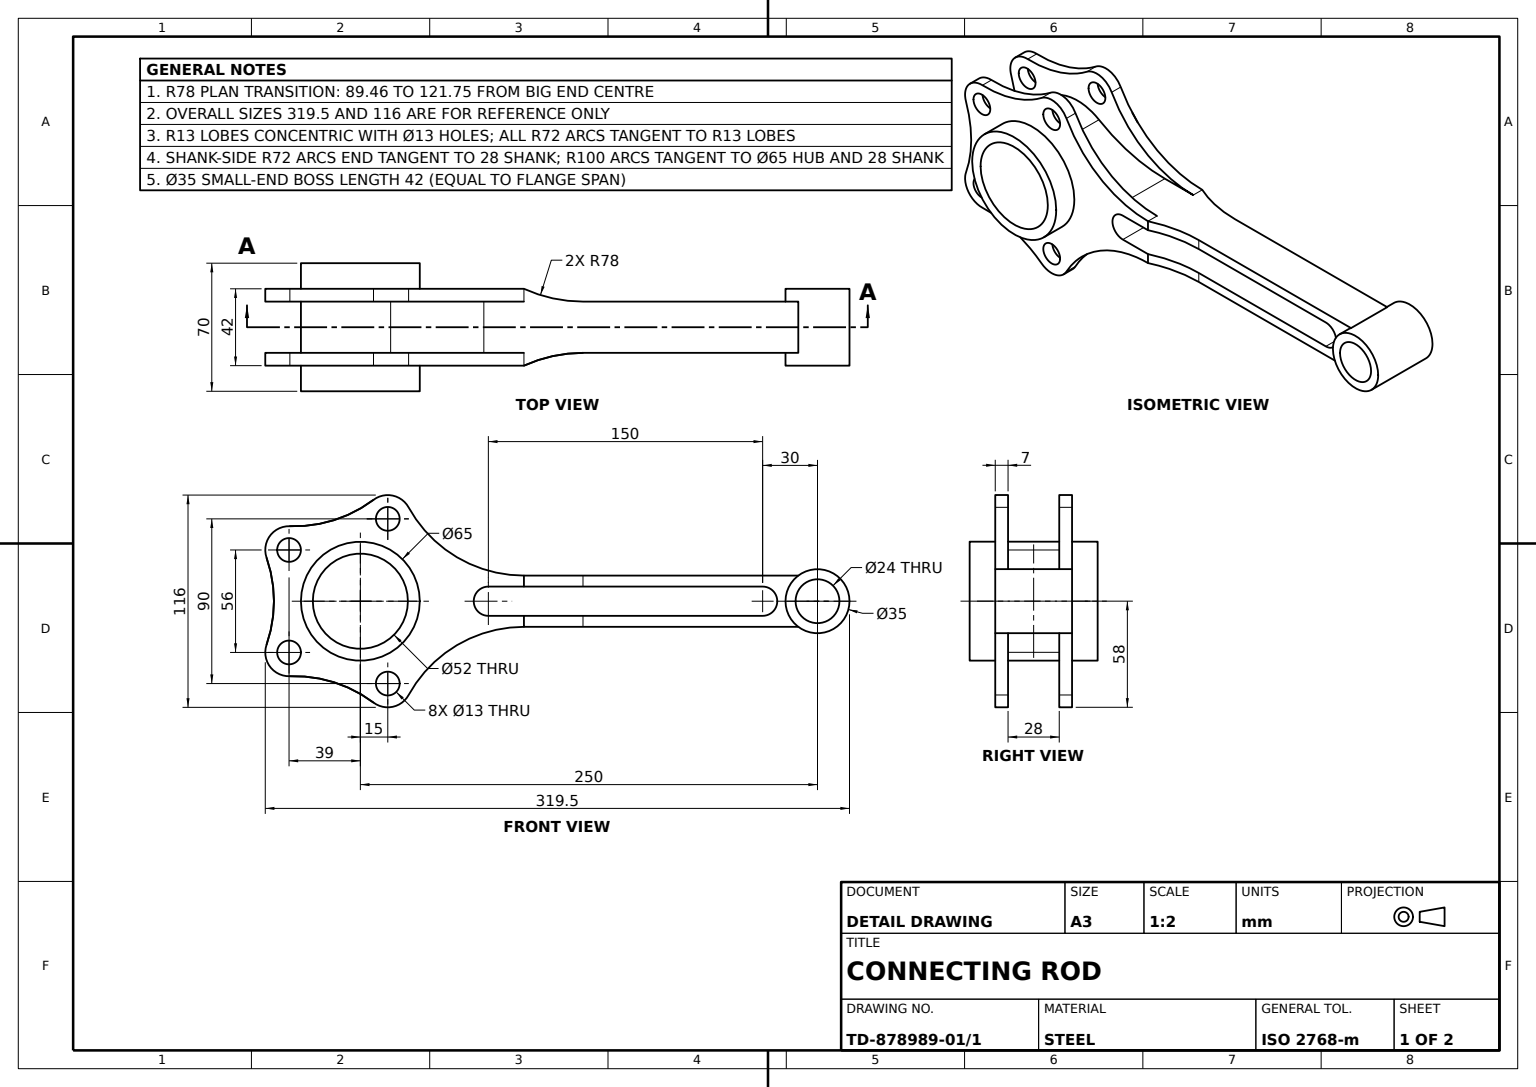
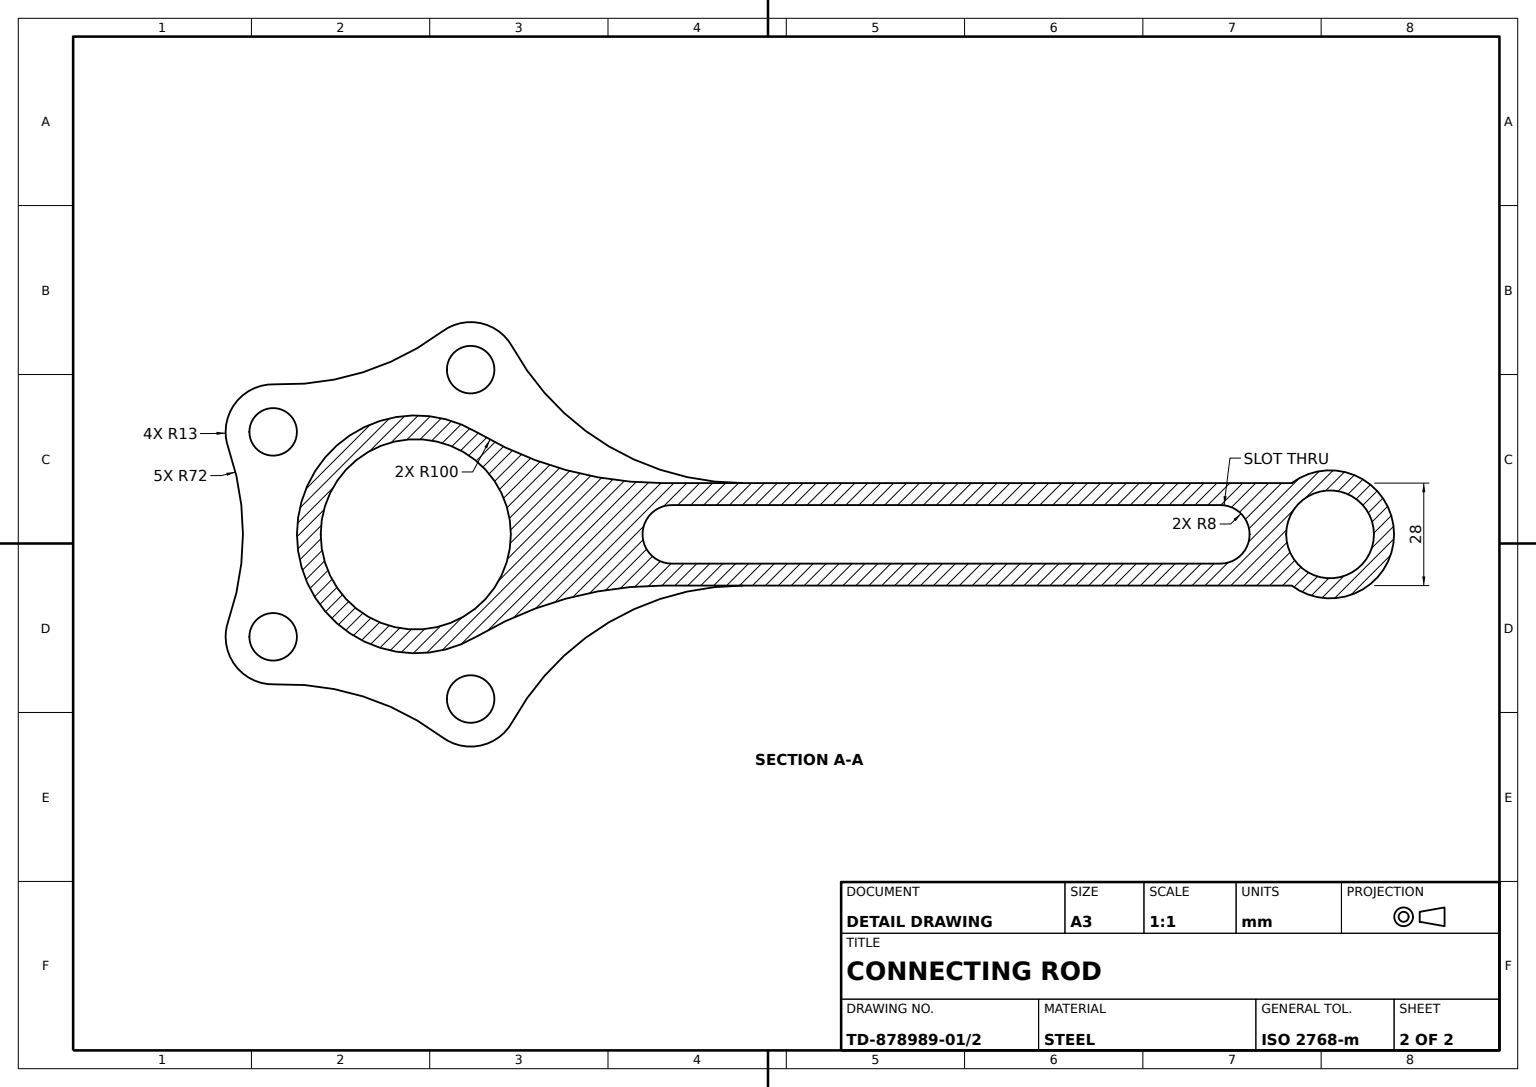
solid
v1 (8.5,-45,14)
v2 (8.5,-45,21)
e1 v1 v2 LINE
v3 (21.5,-45,14)
e2 v1 v3 CIRCLE(AX(P(15,-45,14),D(0,0,-1),D(1,0,0)),6.5)
v4 (21.5,-45,21)
e3 v3 v4 LINE
e4 v2 v4 CIRCLE(AX(P(15,-45,21),D(0,0,-1),D(1,0,0)),6.5)
face CYL(AX(P(15,-45,14),D(0,0,1),D(1,0,0)),6.5) rev [-e1 e2 e3 -e4]
v5 (67.529623,14,14)
v6 (89.458042,14,14)
e5 v5 v6 LINE
v7 (89.458042,14,21)
e6 v6 v7 LINE
v8 (121.753552,14,14)
e7 v7 v8 CIRCLE(AX(P(121.753552,14,92),D(0,-1,0),D(-1,0,0)),78)
v9 (239.5,14,14)
e8 v8 v9 LINE
v10 (239.5,14,-14)
e9 v9 v10 LINE
v11 (121.753552,14,-14)
e10 v11 v10 LINE
v12 (89.458042,14,-21)
e11 v11 v12 CIRCLE(AX(P(121.753552,14,-92),D(0,-1,0),D(-1,0,0)),78)
v13 (89.458042,14,-14)
e12 v13 v12 LINE
v14 (67.529623,14,-14)
e13 v14 v13 LINE
e14 v5 v14 LINE
face PLANE(AX(P(67.529623,14,14),D(0,1,0),D(-1,0,0))) [e5 e6 e7 e8 e9 -e10 e11 -e12 -e13 -e14]
v15 (89.458042,8,-21)
e15 v12 v15 LINE
v16 (121.753552,8,-14)
e16 v16 v11 LINE
e17 v15 v16 CIRCLE(AX(P(121.753552,8,-92),D(0,1,0),D(0,0,1)),78)
face CYL(AX(P(121.753552,14,-92),D(0,1,0),D(0,0,1)),78) rev [-e15 -e11 -e16 -e17]
v17 (8.5,45,14)
v18 (8.5,45,21)
e18 v17 v18 LINE
v19 (21.5,45,21)
e19 v18 v19 CIRCLE(AX(P(15,45,21),D(0,0,1),D(1,0,0)),6.5)
v20 (21.5,45,14)
e20 v20 v19 LINE
e21 v17 v20 CIRCLE(AX(P(15,45,14),D(0,0,1),D(1,0,0)),6.5)
face CYL(AX(P(15,45,14),D(0,0,1),D(1,0,0)),6.5) rev [e18 e19 -e20 -e21]
v21 (-38.551485,40.992261,-21)
v22 (7.189691,55.392261,-21)
e22 v21 v22 CIRCLE(AX(P(-36.067402,112.949396,-21),D(0,0,1),D(1,0,0)),72)
v23 (-38.551485,40.992261,-14)
e23 v23 v21 LINE
v24 (7.189691,55.392261,-14)
e24 v23 v24 CIRCLE(AX(P(-36.067402,112.949396,-14),D(0,0,1),D(1,0,0)),72)
e25 v24 v22 LINE
face CYL(AX(P(-36.067402,112.949396,-14),D(0,0,-1),D(-1,0,0)),72) rev [-e22 -e23 e24 e25]
v25 (-38.551485,-40.992261,14)
v26 (-51.274423,-23.717647,14)
e26 v25 v26 CIRCLE(AX(P(-39,-28,14),D(0,0,-1),D(-1,0,0)),13)
v27 (-38.551485,-40.992261,21)
e27 v25 v27 LINE
v28 (-51.274423,-23.717647,21)
e28 v27 v28 CIRCLE(AX(P(-39,-28,21),D(0,0,-1),D(-1,0,0)),13)
e29 v26 v28 LINE
face CYL(AX(P(-39,-28,14),D(0,0,1),D(1,0,0)),13) [-e26 e27 e28 -e29]
v29 (121.753552,8,14)
v30 (89.458042,8,21)
e30 v29 v30 CIRCLE(AX(P(121.753552,8,92),D(0,1,0),D(0,0,1)),78)
e31 v8 v29 LINE
e32 v7 v30 LINE
face CYL(AX(P(121.753552,14,92),D(0,1,0),D(0,0,1)),78) rev [-e30 -e31 -e7 e32]
v31 (26.387701,-51.270588,14)
v32 (89.458042,-14,14)
e33 v31 v32 CIRCLE(AX(P(89.458042,-86,14),D(0,0,-1),D(-1,0,0)),72)
v33 (7.189691,-55.392261,14)
e34 v31 v33 CIRCLE(AX(P(15,-45,14),D(0,0,-1),D(-1,0,0)),13)
e35 v25 v33 CIRCLE(AX(P(-36.067402,-112.949396,14),D(0,0,-1),D(-1,0,0)),72)
v34 (-47.255841,0,14)
e36 v26 v34 CIRCLE(AX(P(-119.255841,0,14),D(0,0,1),D(1,0,0)),72)
v35 (-51.274423,23.717647,14)
e37 v34 v35 CIRCLE(AX(P(-119.255841,0,14),D(0,0,1),D(1,0,0)),72)
v36 (-38.551485,40.992261,14)
e38 v36 v35 CIRCLE(AX(P(-39,28,14),D(0,0,1),D(1,0,0)),13)
v37 (7.189691,55.392261,14)
e39 v36 v37 CIRCLE(AX(P(-36.067402,112.949396,14),D(0,0,1),D(1,0,0)),72)
v38 (26.387701,51.270588,14)
e40 v38 v37 CIRCLE(AX(P(15,45,14),D(0,0,1),D(1,0,0)),13)
e41 v38 v6 CIRCLE(AX(P(89.458042,86,14),D(0,0,1),D(1,0,0)),72)
v39 (16.56387,27.962264,14)
e42 v39 v5 CIRCLE(AX(P(67.529623,114,14),D(0,0,1),D(1,0,0)),100)
v40 (-32.5,0,14)
e43 v39 v40 CIRCLE(AX(P(0,0,14),D(0,0,1),D(1,0,0)),32.5)
v41 (16.56387,-27.962264,14)
e44 v40 v41 CIRCLE(AX(P(0,0,14),D(0,0,1),D(1,0,0)),32.5)
v42 (67.529623,-14,14)
e45 v41 v42 CIRCLE(AX(P(67.529623,-114,14),D(0,0,-1),D(-1,0,0)),100)
e46 v42 v32 LINE
e47 v20 v17 CIRCLE(AX(P(15,45,14),D(0,0,1),D(1,0,0)),6.5)
v43 (-32.5,28,14)
v44 (-45.5,28,14)
e48 v43 v44 CIRCLE(AX(P(-39,28,14),D(0,0,1),D(1,0,0)),6.5)
e49 v44 v43 CIRCLE(AX(P(-39,28,14),D(0,0,1),D(1,0,0)),6.5)
e50 v3 v1 CIRCLE(AX(P(15,-45,14),D(0,0,-1),D(1,0,0)),6.5)
v45 (-32.5,-28,14)
v46 (-45.5,-28,14)
e51 v45 v46 CIRCLE(AX(P(-39,-28,14),D(0,0,-1),D(1,0,0)),6.5)
e52 v46 v45 CIRCLE(AX(P(-39,-28,14),D(0,0,-1),D(1,0,0)),6.5)
face PLANE(AX(P(-39,28,14),D(0,0,1),D(1,0,0))) rev [-e33 e34 -e35 e26 e36 e37 -e38 e39 -e40 e41 -e5 -e42 e43 e44 e45 e46] [e21 e47] [e48 e49] [-e2 -e50] [-e51 -e52]
v47 (-45.5,28,-21)
v48 (-32.5,28,-21)
e53 v47 v48 CIRCLE(AX(P(-39,28,-21),D(0,0,1),D(1,0,0)),6.5)
e54 v48 v47 CIRCLE(AX(P(-39,28,-21),D(0,0,1),D(1,0,0)),6.5)
v49 (-32.5,-28,-21)
v50 (-45.5,-28,-21)
e55 v49 v50 CIRCLE(AX(P(-39,-28,-21),D(0,0,-1),D(1,0,0)),6.5)
e56 v50 v49 CIRCLE(AX(P(-39,-28,-21),D(0,0,-1),D(1,0,0)),6.5)
v51 (-32.5,0,-21)
v52 (32.5,0,-21)
e57 v51 v52 CIRCLE(AX(P(0,0,-21),D(0,0,-1),D(-1,0,0)),32.5)
e58 v52 v51 CIRCLE(AX(P(0,0,-21),D(0,0,-1),D(-1,0,0)),32.5)
v53 (-52,28,-21)
e59 v21 v53 CIRCLE(AX(P(-39,28,-21),D(0,0,1),D(1,0,0)),13)
v54 (26.387701,51.270588,-21)
e60 v54 v22 CIRCLE(AX(P(15,45,-21),D(0,0,1),D(1,0,0)),13)
e61 v54 v12 CIRCLE(AX(P(89.458042,86,-21),D(0,0,1),D(1,0,0)),72)
v55 (70,8,-21)
e62 v55 v15 LINE
v56 (70,-8,-21)
e63 v56 v55 CIRCLE(AX(P(70,0,-21),D(0,0,-1),D(-1,0,0)),8)
v57 (89.458042,-8,-21)
e64 v57 v56 LINE
v58 (89.458042,-14,-21)
e65 v57 v58 LINE
v59 (26.387701,-51.270588,-21)
e66 v59 v58 CIRCLE(AX(P(89.458042,-86,-21),D(0,0,-1),D(-1,0,0)),72)
v60 (7.189691,-55.392261,-21)
e67 v59 v60 CIRCLE(AX(P(15,-45,-21),D(0,0,-1),D(-1,0,0)),13)
v61 (-38.551485,-40.992261,-21)
e68 v61 v60 CIRCLE(AX(P(-36.067402,-112.949396,-21),D(0,0,-1),D(-1,0,0)),72)
v62 (-52,-28,-21)
e69 v61 v62 CIRCLE(AX(P(-39,-28,-21),D(0,0,-1),D(-1,0,0)),13)
v63 (-51.274423,-23.717647,-21)
e70 v62 v63 CIRCLE(AX(P(-39,-28,-21),D(0,0,-1),D(-1,0,0)),13)
v64 (-51.274423,23.717647,-21)
e71 v63 v64 CIRCLE(AX(P(-119.255841,0,-21),D(0,0,1),D(1,0,0)),72)
e72 v53 v64 CIRCLE(AX(P(-39,28,-21),D(0,0,1),D(1,0,0)),13)
v65 (8.5,-45,-21)
v66 (21.5,-45,-21)
e73 v65 v66 CIRCLE(AX(P(15,-45,-21),D(0,0,-1),D(1,0,0)),6.5)
e74 v66 v65 CIRCLE(AX(P(15,-45,-21),D(0,0,-1),D(1,0,0)),6.5)
v67 (8.5,45,-21)
v68 (21.5,45,-21)
e75 v67 v68 CIRCLE(AX(P(15,45,-21),D(0,0,1),D(1,0,0)),6.5)
e76 v68 v67 CIRCLE(AX(P(15,45,-21),D(0,0,1),D(1,0,0)),6.5)
face PLANE(AX(P(-39,28,-21),D(0,0,-1),D(1,0,0))) [e53 e54] [-e55 -e56] [-e57 -e58] [-e59 e22 -e60 e61 e15 -e62 -e63 -e64 e65 -e66 e67 -e68 e69 e70 e71 -e72] [-e73 -e74] [e75 e76]
v69 (8.5,45,-14)
e77 v69 v67 LINE
v70 (21.5,45,-14)
e78 v70 v68 LINE
e79 v70 v69 CIRCLE(AX(P(15,45,-14),D(0,0,1),D(1,0,0)),6.5)
face CYL(AX(P(15,45,-14),D(0,0,-1),D(-1,0,0)),6.5) rev [e77 -e76 -e78 e79]
v71 (-45.5,28,-14)
e80 v71 v47 LINE
v72 (-32.5,28,-14)
e81 v72 v48 LINE
e82 v72 v71 CIRCLE(AX(P(-39,28,-14),D(0,0,1),D(1,0,0)),6.5)
face CYL(AX(P(-39,28,-14),D(0,0,-1),D(-1,0,0)),6.5) rev [e80 -e54 -e81 e82]
v73 (70,8,21)
e83 v55 v73 LINE
v74 (70,-8,21)
e84 v73 v74 CIRCLE(AX(P(70,0,21),D(0,0,1),D(1,0,0)),8)
e85 v56 v74 LINE
face CYL(AX(P(70,0,-25),D(0,0,1),D(1,0,0)),8) rev [e63 e83 e84 -e85]
v75 (-38.551485,40.992261,21)
v76 (7.189691,55.392261,21)
e86 v75 v76 CIRCLE(AX(P(-36.067402,112.949396,21),D(0,0,1),D(1,0,0)),72)
e87 v37 v76 LINE
e88 v36 v75 LINE
face CYL(AX(P(-36.067402,112.949396,14),D(0,0,1),D(1,0,0)),72) rev [e86 -e87 -e39 e88]
v77 (7.189691,-55.392261,-14)
e89 v77 v60 LINE
v78 (26.387701,-51.270588,-14)
e90 v78 v59 LINE
e91 v78 v77 CIRCLE(AX(P(15,-45,-14),D(0,0,-1),D(-1,0,0)),13)
face CYL(AX(P(15,-45,-14),D(0,0,-1),D(-1,0,0)),13) [e89 -e67 -e90 e91]
v79 (-47.255841,0,21)
e92 v28 v79 CIRCLE(AX(P(-119.255841,0,21),D(0,0,1),D(1,0,0)),72)
v80 (7.189691,-55.392261,21)
e93 v27 v80 CIRCLE(AX(P(-36.067402,-112.949396,21),D(0,0,-1),D(-1,0,0)),72)
v81 (26.387701,-51.270588,21)
e94 v81 v80 CIRCLE(AX(P(15,-45,21),D(0,0,-1),D(-1,0,0)),13)
v82 (89.458042,-14,21)
e95 v81 v82 CIRCLE(AX(P(89.458042,-86,21),D(0,0,-1),D(-1,0,0)),72)
v83 (89.458042,-8,21)
e96 v83 v82 LINE
e97 v74 v83 LINE
e98 v30 v73 LINE
v84 (26.387701,51.270588,21)
e99 v84 v7 CIRCLE(AX(P(89.458042,86,21),D(0,0,1),D(1,0,0)),72)
e100 v84 v76 CIRCLE(AX(P(15,45,21),D(0,0,1),D(1,0,0)),13)
v85 (-51.274423,23.717647,21)
e101 v75 v85 CIRCLE(AX(P(-39,28,21),D(0,0,1),D(1,0,0)),13)
e102 v79 v85 CIRCLE(AX(P(-119.255841,0,21),D(0,0,1),D(1,0,0)),72)
v86 (-32.5,28,21)
v87 (-45.5,28,21)
e103 v86 v87 CIRCLE(AX(P(-39,28,21),D(0,0,1),D(1,0,0)),6.5)
e104 v87 v86 CIRCLE(AX(P(-39,28,21),D(0,0,1),D(1,0,0)),6.5)
v88 (-32.5,0,21)
v89 (32.5,0,21)
e105 v88 v89 CIRCLE(AX(P(0,0,21),D(0,0,1),D(1,0,0)),32.5)
e106 v89 v88 CIRCLE(AX(P(0,0,21),D(0,0,1),D(1,0,0)),32.5)
v90 (-45.5,-28,21)
v91 (-32.5,-28,21)
e107 v90 v91 CIRCLE(AX(P(-39,-28,21),D(0,0,-1),D(1,0,0)),6.5)
e108 v91 v90 CIRCLE(AX(P(-39,-28,21),D(0,0,-1),D(1,0,0)),6.5)
e109 v19 v18 CIRCLE(AX(P(15,45,21),D(0,0,1),D(1,0,0)),6.5)
e110 v4 v2 CIRCLE(AX(P(15,-45,21),D(0,0,-1),D(1,0,0)),6.5)
face PLANE(AX(P(-39,28,21),D(0,0,1),D(1,0,0))) [-e92 -e28 e93 -e94 e95 -e96 -e97 -e84 -e98 -e32 -e99 e100 -e86 e101 -e102] [-e103 -e104] [-e105 -e106] [e107 e108] [-e109 -e19] [e110 e4]
e111 v44 v87 LINE
e112 v43 v86 LINE
face CYL(AX(P(-39,28,14),D(0,0,1),D(1,0,0)),6.5) rev [e103 -e111 -e48 e112]
v92 (238,0,21)
v93 (262,0,21)
e113 v92 v93 CIRCLE(AX(P(250,0,21),D(0,0,1),D(1,0,0)),12)
v94 (262,0,-21)
e114 v93 v94 LINE
v95 (238,0,-21)
e115 v95 v94 CIRCLE(AX(P(250,0,-21),D(0,0,1),D(1,0,0)),12)
e116 v92 v95 LINE
face CYL(AX(P(250,0,21),D(0,0,-1),D(-1,0,0)),12) rev [e113 e114 -e115 -e116]
v96 (-52,28,-14)
v97 (-51.274423,23.717647,-14)
e117 v96 v97 CIRCLE(AX(P(-39,28,-14),D(0,0,1),D(1,0,0)),13)
e118 v96 v53 LINE
e119 v97 v64 LINE
face CYL(AX(P(-39,28,-14),D(0,0,-1),D(-1,0,0)),13) [-e117 e118 e72 -e119]
v98 (-32.5,0,35)
v99 (32.5,0,35)
e120 v98 v99 CIRCLE(AX(P(0,0,35),D(0,0,1),D(1,0,0)),32.5)
e121 v99 v98 CIRCLE(AX(P(0,0,35),D(0,0,1),D(1,0,0)),32.5)
v100 (26,0,35)
v101 (-26,0,35)
e122 v100 v101 CIRCLE(AX(P(0,0,35),D(0,0,1),D(1,0,0)),26)
e123 v101 v100 CIRCLE(AX(P(0,0,35),D(0,0,1),D(1,0,0)),26)
face PLANE(AX(P(0,0,35),D(0,0,1),D(1,0,0))) [e120 e121] [-e122 -e123]
v102 (220,8,-14)
e124 v102 v16 LINE
v103 (220,8,14)
e125 v102 v103 LINE
e126 v103 v29 LINE
face PLANE(AX(P(70,8,-25),D(0,1,0),D(0,0,1))) rev [e17 -e124 e125 e126 e30 e98 -e83 e62]
v104 (228,0,-14)
e127 v104 v102 CIRCLE(AX(P(220,0,-14),D(0,0,1),D(1,0,0)),8)
v105 (228,0,14)
e128 v104 v105 LINE
e129 v105 v103 CIRCLE(AX(P(220,0,14),D(0,0,1),D(1,0,0)),8)
face CYL(AX(P(220,0,-25),D(0,0,1),D(1,0,0)),8) rev [-e125 -e127 e128 e129]
v106 (121.753552,-8,-14)
e130 v106 v57 CIRCLE(AX(P(121.753552,-8,-92),D(0,-1,0),D(0,0,-1)),78)
v107 (121.753552,-14,-14)
e131 v107 v106 LINE
e132 v58 v107 CIRCLE(AX(P(121.753552,-14,-92),D(0,1,0),D(-1,0,0)),78)
face CYL(AX(P(121.753552,14,-92),D(0,1,0),D(0,0,1)),78) rev [-e65 -e130 -e131 -e132]
v108 (-51.274423,-23.717647,-14)
e133 v108 v97 CIRCLE(AX(P(-119.255841,0,-14),D(0,0,1),D(1,0,0)),72)
e134 v108 v63 LINE
face CYL(AX(P(-119.255841,0,-14),D(0,0,-1),D(-1,0,0)),72) rev [e133 e119 -e71 -e134]
e135 v98 v88 LINE
e136 v99 v89 LINE
face CYL(AX(P(0,0,35),D(0,0,-1),D(-1,0,0)),32.5) [-e135 -e121 e136 e106]
v109 (239.5,-14,-14)
e137 v107 v109 LINE
v110 (239.5,-14,14)
e138 v110 v109 LINE
v111 (121.753552,-14,14)
e139 v111 v110 LINE
e140 v111 v82 CIRCLE(AX(P(121.753552,-14,92),D(0,1,0),D(-1,0,0)),78)
e141 v32 v82 LINE
v112 (67.529623,-14,-14)
e142 v42 v112 LINE
v113 (89.458042,-14,-14)
e143 v112 v113 LINE
e144 v113 v58 LINE
face PLANE(AX(P(67.529623,-14,14),D(0,1,0),D(-1,0,0))) rev [e137 -e138 -e139 e140 -e141 -e46 e142 e143 e144 e132]
v114 (121.753552,-8,14)
e145 v114 v111 LINE
e146 v83 v114 CIRCLE(AX(P(121.753552,-8,92),D(0,-1,0),D(0,0,-1)),78)
face CYL(AX(P(121.753552,14,92),D(0,1,0),D(0,0,1)),78) rev [-e145 -e146 e96 -e140]
v115 (220,-8,-14)
e147 v115 v104 CIRCLE(AX(P(220,0,-14),D(0,0,1),D(1,0,0)),8)
v116 (220,-8,14)
e148 v115 v116 LINE
e149 v116 v105 CIRCLE(AX(P(220,0,14),D(0,0,1),D(1,0,0)),8)
face CYL(AX(P(220,0,-25),D(0,0,1),D(1,0,0)),8) rev [-e147 e148 e149 -e128]
e150 v45 v91 LINE
e151 v46 v90 LINE
face CYL(AX(P(-39,-28,14),D(0,0,1),D(1,0,0)),6.5) rev [e150 -e107 -e151 e52]
e152 v93 v92 CIRCLE(AX(P(250,0,21),D(0,0,1),D(1,0,0)),12)
v117 (267.5,0,21)
v118 (232.5,0,21)
e153 v117 v118 CIRCLE(AX(P(250,0,21),D(0,0,1),D(1,0,0)),17.5)
e154 v118 v117 CIRCLE(AX(P(250,0,21),D(0,0,1),D(1,0,0)),17.5)
face PLANE(AX(P(250,0,21),D(0,0,1),D(1,0,0))) [-e113 -e152] [e153 e154]
v119 (-32.5,0,-35)
v120 (32.5,0,-35)
e155 v119 v120 CIRCLE(AX(P(0,0,-35),D(0,0,1),D(1,0,0)),32.5)
e156 v120 v119 CIRCLE(AX(P(0,0,-35),D(0,0,1),D(1,0,0)),32.5)
v121 (-26,0,-35)
v122 (26,0,-35)
e157 v121 v122 CIRCLE(AX(P(0,0,-35),D(0,0,1),D(1,0,0)),26)
e158 v122 v121 CIRCLE(AX(P(0,0,-35),D(0,0,1),D(1,0,0)),26)
face PLANE(AX(P(0,0,-35),D(0,0,1),D(1,0,0))) rev [-e155 -e156] [e157 e158]
e159 v51 v119 LINE
e160 v52 v120 LINE
face CYL(AX(P(0,0,35),D(0,0,-1),D(-1,0,0)),32.5) [e156 -e159 e57 e160]
e161 v94 v95 CIRCLE(AX(P(250,0,-21),D(0,0,1),D(1,0,0)),12)
face CYL(AX(P(250,0,21),D(0,0,-1),D(-1,0,0)),12) rev [e152 e116 -e161 -e114]
v123 (26.387701,51.270588,-14)
e162 v123 v54 LINE
e163 v123 v13 CIRCLE(AX(P(89.458042,86,-14),D(0,0,1),D(1,0,0)),72)
face CYL(AX(P(89.458042,86,-14),D(0,0,-1),D(-1,0,0)),72) rev [e12 -e61 -e162 e163]
face CYL(AX(P(-39,28,14),D(0,0,1),D(1,0,0)),6.5) rev [-e112 -e49 e111 e104]
v124 (232.5,0,14)
e164 v118 v124 LINE
e165 v124 v110 CIRCLE(AX(P(250,0,14),D(0,0,1),D(1,0,0)),17.5)
v125 (232.5,0,-14)
e166 v125 v109 CIRCLE(AX(P(250,0,-14),D(0,0,1),D(1,0,0)),17.5)
v126 (232.5,0,-21)
e167 v125 v126 LINE
v127 (267.5,0,-21)
e168 v126 v127 CIRCLE(AX(P(250,0,-21),D(0,0,1),D(1,0,0)),17.5)
e169 v117 v127 LINE
face CYL(AX(P(250,0,21),D(0,0,-1),D(-1,0,0)),17.5) [-e154 e164 e165 e138 -e166 e167 e168 -e169]
e170 v69 v70 CIRCLE(AX(P(15,45,-14),D(0,0,1),D(1,0,0)),6.5)
face CYL(AX(P(15,45,-14),D(0,0,-1),D(-1,0,0)),6.5) rev [-e77 e170 e78 -e75]
v128 (-52,-28,-14)
e171 v128 v108 CIRCLE(AX(P(-39,-28,-14),D(0,0,-1),D(-1,0,0)),13)
e172 v128 v62 LINE
face CYL(AX(P(-39,-28,-14),D(0,0,-1),D(-1,0,0)),13) [e171 e134 -e70 -e172]
v129 (16.56387,27.962264,-14)
e173 v39 v129 LINE
v130 (-32.5,0,-14)
e174 v130 v129 CIRCLE(AX(P(0,0,-14),D(0,0,-1),D(-1,0,0)),32.5)
e175 v40 v130 LINE
face CYL(AX(P(0,0,35),D(0,0,-1),D(-1,0,0)),32.5) [e173 -e174 -e175 -e43]
e176 v129 v14 CIRCLE(AX(P(67.529623,114,-14),D(0,0,1),D(1,0,0)),100)
face CYL(AX(P(67.529623,114,14),D(0,0,-1),D(-1,0,0)),100) rev [e42 e14 -e176 -e173]
e177 v114 v116 LINE
e178 v9 v124 CIRCLE(AX(P(250,0,14),D(0,0,1),D(1,0,0)),17.5)
face PLANE(AX(P(67.529623,114,14),D(0,0,1),D(1,0,0))) [e31 -e126 -e129 -e149 -e177 e145 e139 -e165 -e178 -e8]
e179 v101 v121 LINE
e180 v100 v122 LINE
face CYL(AX(P(0,0,35),D(0,0,-1),D(-1,0,0)),26) rev [-e179 e123 e180 -e157]
face CYL(AX(P(-39,-28,14),D(0,0,1),D(1,0,0)),6.5) rev [-e150 e51 e151 -e108]
face CYL(AX(P(15,45,14),D(0,0,1),D(1,0,0)),6.5) rev [-e47 e20 e109 -e18]
v131 (-45.5,-28,-14)
e181 v131 v50 LINE
v132 (-32.5,-28,-14)
e182 v132 v131 CIRCLE(AX(P(-39,-28,-14),D(0,0,-1),D(1,0,0)),6.5)
e183 v132 v49 LINE
face CYL(AX(P(-39,-28,-14),D(0,0,-1),D(-1,0,0)),6.5) rev [-e181 -e182 e183 e55]
e184 v123 v24 CIRCLE(AX(P(15,45,-14),D(0,0,1),D(1,0,0)),13)
face CYL(AX(P(15,45,-14),D(0,0,-1),D(-1,0,0)),13) [-e25 -e184 e162 e60]
v133 (8.5,-45,-14)
e185 v133 v65 LINE
v134 (21.5,-45,-14)
e186 v134 v133 CIRCLE(AX(P(15,-45,-14),D(0,0,-1),D(1,0,0)),6.5)
e187 v134 v66 LINE
face CYL(AX(P(15,-45,-14),D(0,0,-1),D(-1,0,0)),6.5) rev [-e185 -e186 e187 e74]
e188 v106 v115 LINE
face PLANE(AX(P(70,-8,-25),D(0,-1,0),D(0,0,-1))) rev [e97 e146 e177 -e148 -e188 e130 e64 e85]
v135 (-38.551485,-40.992261,-14)
e189 v135 v61 LINE
e190 v135 v128 CIRCLE(AX(P(-39,-28,-14),D(0,0,-1),D(-1,0,0)),13)
face CYL(AX(P(-39,-28,-14),D(0,0,-1),D(-1,0,0)),13) [-e189 e190 e172 -e69]
face CYL(AX(P(15,-45,14),D(0,0,1),D(1,0,0)),6.5) rev [e50 e1 -e110 -e3]
e191 v38 v84 LINE
face CYL(AX(P(15,45,14),D(0,0,1),D(1,0,0)),13) [e87 -e100 -e191 e40]
e192 v31 v81 LINE
face CYL(AX(P(89.458042,-86,14),D(0,0,1),D(1,0,0)),72) rev [-e192 e33 e141 -e95]
e193 v33 v80 LINE
face CYL(AX(P(15,-45,14),D(0,0,1),D(1,0,0)),13) [e94 -e193 -e34 e192]
face CYL(AX(P(-36.067402,-112.949396,14),D(0,0,1),D(1,0,0)),72) rev [e35 e193 -e93 -e27]
e194 v34 v79 LINE
face CYL(AX(P(-119.255841,0,14),D(0,0,1),D(1,0,0)),72) rev [e29 e92 -e194 -e36]
face CYL(AX(P(0,0,35),D(0,0,-1),D(-1,0,0)),32.5) [-e160 e58 e159 e155]
e195 v35 v85 LINE
face CYL(AX(P(-119.255841,0,14),D(0,0,1),D(1,0,0)),72) rev [-e195 -e37 e194 e102]
e196 v135 v77 CIRCLE(AX(P(-36.067402,-112.949396,-14),D(0,0,-1),D(-1,0,0)),72)
face CYL(AX(P(-36.067402,-112.949396,-14),D(0,0,-1),D(-1,0,0)),72) rev [-e89 -e196 e189 e68]
face CYL(AX(P(0,0,35),D(0,0,-1),D(-1,0,0)),32.5) [-e120 e135 e105 -e136]
e197 v23 v96 CIRCLE(AX(P(-39,28,-14),D(0,0,1),D(1,0,0)),13)
face CYL(AX(P(-39,28,-14),D(0,0,-1),D(-1,0,0)),13) [-e197 e23 e59 -e118]
e198 v133 v134 CIRCLE(AX(P(15,-45,-14),D(0,0,-1),D(1,0,0)),6.5)
face CYL(AX(P(15,-45,-14),D(0,0,-1),D(-1,0,0)),6.5) rev [-e187 -e198 e185 e73]
v136 (16.56387,-27.962264,-14)
e199 v136 v112 CIRCLE(AX(P(67.529623,-114,-14),D(0,0,-1),D(-1,0,0)),100)
e200 v41 v136 LINE
face CYL(AX(P(67.529623,-114,14),D(0,0,-1),D(-1,0,0)),100) rev [e199 -e142 -e45 e200]
e201 v78 v113 CIRCLE(AX(P(89.458042,-86,-14),D(0,0,-1),D(-1,0,0)),72)
face CYL(AX(P(89.458042,-86,-14),D(0,0,-1),D(-1,0,0)),72) rev [-e144 -e201 e90 e66]
face CYL(AX(P(0,0,35),D(0,0,-1),D(-1,0,0)),26) rev [-e180 e122 e179 -e158]
e202 v71 v72 CIRCLE(AX(P(-39,28,-14),D(0,0,1),D(1,0,0)),6.5)
face CYL(AX(P(-39,28,-14),D(0,0,-1),D(-1,0,0)),6.5) rev [e81 -e53 -e80 e202]
face CYL(AX(P(-39,28,14),D(0,0,1),D(1,0,0)),13) [e195 -e101 -e88 e38]
e203 v127 v126 CIRCLE(AX(P(250,0,-21),D(0,0,1),D(1,0,0)),17.5)
e204 v10 v125 CIRCLE(AX(P(250,0,-14),D(0,0,1),D(1,0,0)),17.5)
face CYL(AX(P(250,0,21),D(0,0,-1),D(-1,0,0)),17.5) [e178 -e164 -e153 e169 e203 -e167 -e204 -e9]
e205 v131 v132 CIRCLE(AX(P(-39,-28,-14),D(0,0,-1),D(1,0,0)),6.5)
e206 v136 v130 CIRCLE(AX(P(0,0,-14),D(0,0,-1),D(-1,0,0)),32.5)
face PLANE(AX(P(-39,28,-14),D(0,0,-1),D(1,0,0))) rev [e182 e205] [e196 -e91 e201 -e143 -e199 e206 e174 e176 e13 -e163 e184 -e24 e197 e117 -e133 -e171 -e190] [-e82 -e202] [-e79 -e170] [e198 e186]
face CYL(AX(P(-39,-28,-14),D(0,0,-1),D(-1,0,0)),6.5) rev [-e205 e181 e56 -e183]
face PLANE(AX(P(250,0,-21),D(0,0,1),D(1,0,0))) rev [e161 e115] [-e168 -e203]
face PLANE(AX(P(67.529623,114,-14),D(0,0,1),D(1,0,0))) rev [-e137 e131 e188 e147 e127 e124 e16 e10 e204 e166]
face CYL(AX(P(89.458042,86,14),D(0,0,1),D(1,0,0)),72) rev [-e6 -e41 e191 e99]
face CYL(AX(P(0,0,35),D(0,0,-1),D(-1,0,0)),32.5) [-e206 -e200 -e44 e175]
